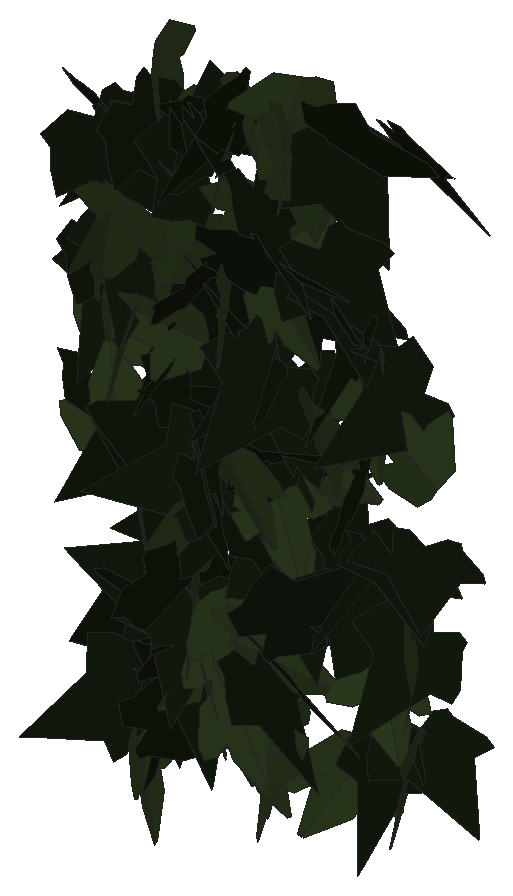
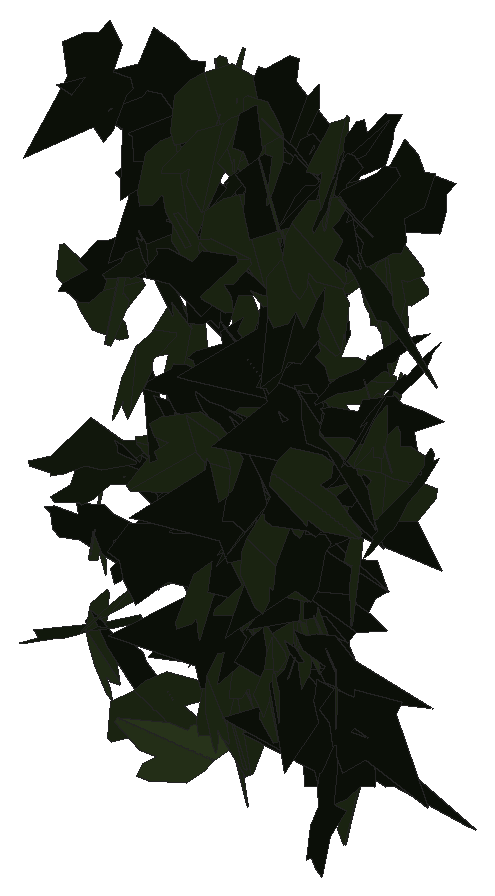
# SketchUp Ruby script. Lengths in inches.
U = 1.inch
M = Sketchup.active_model
def pt(a) = Geom::Point3d.new(a.map { |v| v * U })
def face(e, loops, mat)
  f = e.add_face(loops[0].map { |a| pt(a) })
  loops[1..].each { |l| e.add_face(l.map { |a| pt(a) }).erase! }
  f.material = f.back_material = mat if mat
  f
end
# faces: each face lists its corners as indices into pts; further lists are holes
def faces(e, pts, list, mat = nil) = list.each { |f| face(e, (f[0].is_a?(Array) ? f : [f]).map { |l| l.map { |i| pts[i] } }, mat) }
# xy, xz, yz: faces in a plane at the given z, y or x. An outline is a flat list of corners, or four numbers for a rectangle; further outlines are holes
def ring(l) = l.size == 4 ? [[l[0], l[1]], [l[2], l[1]], [l[2], l[3]], [l[0], l[3]]] : l.each_slice(2).to_a
def flat(e, list, mat, &to3) = list.each { |f| face(e, (f[0].is_a?(Array) ? f : [f]).map { |l| ring(l).map { |u, v| to3.(u, v) } }, mat) }
def xy(e, z, list, mat = nil) = flat(e, list, mat) { |x, y| [x, y, z] }
def xz(e, y, list, mat = nil) = flat(e, list, mat) { |x, z| [x, y, z] }
def yz(e, x, list, mat = nil) = flat(e, list, mat) { |y, z| [x, y, z] }
def lines(e, pts, list) = list.each { |a, b| e.add_line(pt(pts[a]), pt(pts[b])) }
# prism: a flat outline (further loops are holes) pulled along v
def prism(e, loops, v, mat = nil)
  f = face(e, loops, mat); d = Geom::Vector3d.new(v.map { |x| x * U })
  f.pushpull(f.normal.samedirection?(d) ? d.length : -d.length)
end
def box(e, o, s, mat = nil) = prism(e, [[o, [o[0] + s[0], o[1], o[2]], [o[0] + s[0], o[1] + s[1], o[2]], [o[0], o[1] + s[1], o[2]]]], [0, 0, s[2]], mat)
def at(x, y, z, deg = 0) = Geom::Transformation.translation(pt([x, y, z])) * Geom::Transformation.rotation(ORIGIN, Z_AXIS, deg.degrees)
def axes(o, x, y, z) = Geom::Transformation.new([*x, 0, *y, 0, *z, 0, *pt(o).to_a, 1])
def part(name) = M.definitions.add(name)
# library, detail: a bought-in or finely detailed component or shape, given as its bounding box
def library(name, o, s) = part(name).tap { |d| box(d.entities, o, s) }
def detail(e, o, s) = box(e.add_group.entities, o, s)
def put(e, d, t, mat = nil) = e.add_instance(d, t).tap { |i| i.material = mat if mat }
def group(e, t, mat = nil) = e.add_group.tap { |g| g.transformation = t; g.material = mat if mat }.entities
root = M.entities
M.materials.add("efeu1").color = [18, 25, 13]
M.materials.add("efeu2").color = [43, 57, 29]
c1 = part("ivyleaf_9")
p = [[1.54,2.16,1.25],[1.36,2.04,1.19],[-0.21,0.99,0.68],[-0.71,1.11,0.82],[-0.85,0.86,0.67],[-0.8,0.17,0.21],
  [-0.9,-0.01,0.1],[-0.67,-0.16,-0.02],[-0.08,-0.08,-0.05],[-0.03,-0.6,-0.4],[0.65,-0.88,-0.66],[0.83,-0.6,-0.49],
  [1.29,-0.42,-0.43],[1.8125,-0.07,-0.26],[1.21,0.44,0.15]]
faces(c1.entities,p,[[0,1,2,3,4,5,6,7,8,9,10,11,12,13,14]],"efeu1")
c2 = part("ivyleaf_10")
p = [[0,0.5,-0.03],[-0.0625,2.02,-0.43],[-0.19,2.01,-0.46],[-0.54,1.05,-0.29],[-0.52,0.625,-0.18],[-0.83,0.76,-0.28],
  [-1.16,0.64,-0.33],[-1.15,0.33,-0.24],[-0.77,-0.39,0.02],[-0.3,-0.51,0.16],[0.04,-0.48,0.23],[-0.02,2.01,-0.4375],
  [-0.06,2.01,-0.43],[0.04,-0.49,0.23],[0.67,-0.49,0.14],[1.38,0.36,-0.2],[1.375,0.51,-0.24],[0.81,0.65,-0.19],
  [0.62,0.59,-0.15],[0.6,1.09,-0.28],[0.5,1.23,-0.31]]
faces(c2.entities,p,[[0,1,2,3,4,5,6,7,8,9,10],[11,12,0,13,14,15,16,17,18,19,20]],"efeu2")
put(root,c1,axes([46.8,220.97,240.32],[0.3865,-0.05455,0.31248],[0.31369,-0.00741,-0.38929],[0.0471,0.49696,0.0285]))
put(root,c1,axes([46.45,221.32,237.34],[-0.37233,-0.02297,0.33293],[-0.32073,-0.11324,-0.36649],[0.09223,-0.48647,0.06959]))
put(root,c2,axes([45.4,221.08,240.3],[-0.46109,-0.04072,0.18904],[-0.18522,-0.04747,-0.462],[0.05558,-0.49607,0.02869]))
put(root,c1,axes([47.14,221.15,235.26],[0.24333,-0.42307,-0.10864],[-0.00438,0.12198,-0.48487],[0.43677,0.23692,0.05565]))
put(root,c1,axes([47.59,220.82,236.08],[0.04335,-0.00485,0.49809],[0.43952,0.23565,-0.03596],[-0.23441,0.44096,0.02469]))
put(root,c2,axes([46.95,221.07,237.77],[-0.45451,0.15093,-0.14368],[0.13832,-0.03931,-0.47887],[-0.15585,-0.47505,-0.00602]))
put(root,c1,axes([45.6,220.99,241.68],[0.15793,-0.2727,-0.38819],[-0.19318,0.33671,-0.31513],[0.43329,0.24952,0.001]))
put(root,c2,axes([46.45,221.12,235.07],[-0.28638,0.40461,-0.06538],[0.04195,-0.0504,-0.49568],[-0.40771,-0.28939,-0.00508]))
put(root,c2,axes([45.11,221.16,240.08],[0.05069,-0.48393,-0.11506],[-0.00378,0.11528,-0.48651],[0.49741,0.05019,0.00802]))
put(root,c2,axes([47.09,221.34,234.12],[0.22014,-0.15433,-0.42157],[0.35015,-0.23481,0.26881],[-0.28095,-0.41358,0.0047]))
put(root,c1,axes([46.64,221.52,241.95],[-0.16242,0.05528,-0.46964],[0.24306,-0.4162,-0.13305],[-0.40563,-0.27152,0.10833]))
put(root,c2,axes([46.91,221.08,234.8],[0.20428,0.43228,0.14629],[0.06712,0.13007,-0.4781],[-0.4514,0.21497,-0.00489]))
put(root,c1,axes([47.12,221.55,238.77],[-0.27886,-0.37937,0.16826],[-0.10219,-0.13371,-0.47083],[0.40224,-0.29698,-0.00296]))
put(root,c1,axes([46.08,221.39,235.74],[-0.32828,-0.32936,-0.18372],[0.13373,0.12609,-0.46499],[0.35263,-0.35444,0.00531]))
put(root,c2,axes([46.48,221.46,239.78],[0.21073,-0.29148,0.34732],[0.2627,-0.23369,-0.3555],[0.36957,0.33231,0.05465]))
put(root,c1,axes([48.99,221.6,239.09],[-0.26032,-0.30662,0.29702],[-0.19163,-0.22693,-0.40222],[0.38146,-0.32325,0.00064]))
put(root,c1,axes([46.98,221.33,240.98],[0.28987,-0.40717,-0.01377],[-0.00797,0.01123,-0.49981],[0.40732,0.28998,0.00001]))
put(root,c1,axes([45,221.09,241.28],[-0.0026,-0.26845,-0.42182],[0.01219,0.42166,-0.26842],[0.49984,-0.01168,0.00435]))
put(root,c2,axes([45.51,221.24,233.6875],[-0.13103,0.47752,-0.0693],[0.01853,-0.06678,-0.49517],[-0.48217,-0.13234,-0.0002]))
put(root,c2,axes([49.36,221.24,238.45],[0.27981,0.08174,0.40623],[-0.40276,-0.06157,0.28982],[0.0974,-0.48942,0.03139]))
put(root,c1,axes([45.51,221.43,237.51],[0.04991,0.09928,-0.48749],[-0.23004,-0.42982,-0.11109],[-0.44113,0.23537,0.00277]))
put(root,c2,axes([45.97,221.55,235.625],[0.18684,-0.17763,0.42842],[0.31477,-0.29063,-0.25778],[0.3406,0.36603,0.00322]))
put(root,c2,axes([46.27,221.24,236.95],[-0.11995,-0.47387,-0.10515],[0.02458,0.10224,-0.48882],[0.48478,-0.12244,-0.00123]))
put(root,c1,axes([45.9,220.89,236.13],[-0.01835,0.1511,-0.47627],[-0.10473,0.46484,0.15151],[0.48856,0.10532,0.01459]))
put(root,c2,axes([47.08,221.33,234.27],[-0.44844,0.04095,-0.21731],[-0.21722,0.01045,0.45023],[0.04141,0.49821,0.00842]))
put(root,c2,axes([45.18,221.39,238.78],[0.28611,-0.40895,0.03005],[0.01789,-0.02416,-0.4991],[0.40966,0.28667,0.0008]))
put(root,c1,axes([46,221.41,237.5625],[-0.13717,-0.06246,-0.47674],[0.46737,0.09909,-0.14746],[0.1129,-0.48609,0.0312]))
put(root,c1,axes([46.26,221.26,241.59],[0.42677,-0.24662,-0.08393],[-0.06824,0.04963,-0.49283],[0.25142,0.4321,0.0087]))
put(root,c1,axes([44.72,221.45,241.19],[0.27844,-0.27235,0.31351],[0.2605,-0.17942,-0.38723],[0.32343,0.37899,0.04198]))
put(root,c2,axes([47.47,221.17,241.82],[0.25936,-0.28035,-0.32271],[-0.15566,0.2896,-0.37669],[0.39812,0.29586,0.06294]))
put(root,c1,axes([46.25,221.24,237.4375],[0.31981,-0.27864,-0.26473],[-0.1758,0.2002,-0.4231],[0.34178,0.3637,0.03009]))
put(root,c2,axes([46.64,221.31,235.36],[0.32468,0.37426,0.06716],[0.04255,0.05199,-0.49547],[-0.37785,0.32745,0.00191]))
put(root,c1,axes([46.01,221.61,240.8],[-0.04527,-0.4943,-0.06015],[0.05638,-0.0651,0.49253],[-0.49474,0.03781,0.06163]))
put(root,c2,axes([46.62,221.31,235.74],[0.20407,0.45593,0.02201],[0.01219,0.01865,-0.4995],[-0.4563,0.2044,-0.0035]))
put(root,c1,axes([45.18,221.47,234.19],[-0.46648,0.07003,0.16582],[-0.16471,0.01968,-0.47168],[-0.07259,-0.49468,0.00471]))
put(root,c2,axes([46.28,221.6875,235.01],[0.01666,0.21113,-0.45293],[-0.1853,-0.41826,-0.20179],[-0.4641,0.17458,0.06431]))
put(root,c1,axes([46.01,221.47,234.94],[-0.28027,-0.15592,-0.38358],[0.34576,0.16671,-0.3204],[0.22781,-0.44486,0.01437]))
put(root,c1,axes([46.38,221.38,236.81],[-0.40019,0.19108,0.23094],[-0.21769,0.07954,-0.44304],[-0.20605,-0.45515,0.01953]))
put(root,c1,axes([45.76,221.09,234.12],[0.15187,0.07913,0.46976],[0.4243,0.2017,-0.17115],[-0.21658,0.45062,-0.00588]))
put(root,c2,axes([47.89,221.31,238.53],[-0.46044,0.18598,0.05835],[-0.05402,0.02207,-0.49658],[-0.18729,-0.4636,-0.00023]))
put(root,c2,axes([47.25,221.58,241.38],[-0.2165,0.36448,0.26511],[0.12921,-0.23157,0.42389],[0.43178,0.25205,0.00608]))
put(root,c2,axes([47.05,221.61,235.58],[-0.23287,-0.32846,0.29645],[-0.16387,-0.24715,-0.40257],[0.41099,-0.28465,0.00746]))
put(root,c2,axes([45.04,221.35,237.36],[0.38861,0.31443,0.01081],[-0.01058,-0.0041,0.49987],[0.31443,-0.38874,0.00347]))
put(root,c2,axes([45.47,221.26,236.81],[-0.23988,0.38309,0.21378],[-0.18833,0.13013,-0.44452],[-0.39622,-0.29378,0.08186]))
put(root,c2,axes([46.98,221.4,235.37],[-0.16905,0.01972,-0.47014],[0.47032,-0.00867,-0.16948],[-0.01484,-0.49954,-0.01562]))
put(root,c1,axes([47.02,221.46,235.25],[0.4307,-0.21881,0.12891],[0.11656,-0.05517,-0.48308],[0.22563,0.44618,0.00348]))
put(root,c1,axes([44.51,221.64,237.69],[0.22848,-0.43045,0.11183],[0.06616,-0.09143,-0.4871],[0.43979,0.23738,0.01518]))
put(root,c2,axes([47.12,221.45,237.28],[0.43584,0.12416,0.21125],[0.20167,0.06311,-0.45315],[-0.13919,0.48021,0.00494]))
put(root,c2,axes([46.28,221.4,235.5],[-0.48934,0.05727,0.08524],[-0.08591,-0.00088,-0.49256],[-0.05627,-0.49671,0.0107]))
put(root,c2,axes([45.98,221.6,240.08],[-0.24076,-0.39503,0.18971],[-0.10624,-0.15739,-0.46254],[0.42515,-0.26303,-0.00815]))
put(root,c2,axes([47.09,221.52,233.97],[0.33007,-0.37391,-0.03533],[-0.00901,0.03914,-0.49838],[0.37546,0.32964,0.0191]))
put(root,c1,axes([47.02,221.53,238.86],[-0.45965,0.19027,-0.05021],[0.04713,-0.01742,-0.49747],[-0.19105,-0.46206,-0.00192]))
put(root,c2,axes([45.86,221.5,238.78],[-0.08838,0.00362,-0.49211],[-0.49051,0.03991,0.08838],[0.03992,0.49839,-0.0035]))
put(root,c1,axes([46.21,221.11,239.66],[0.15741,0.43259,0.19515],[0.0444,0.19128,-0.45983],[-0.47249,0.1621,0.02181]))
put(root,c1,axes([48.2,221.62,239.65],[-0.39666,0.1439,-0.26824],[0.24774,-0.10338,-0.42182],[-0.17686,-0.46755,0.01072]))
put(root,c1,axes([46.3,221.4,241.39],[-0.31342,0.2725,0.27841],[-0.22956,0.15952,-0.41456],[-0.31476,-0.38768,0.02512]))
put(root,c1,axes([46.12,221.27,235.16],[0.19447,0.45928,-0.03522],[-0.01608,-0.03144,-0.49875],[-0.46035,0.19511,0.00254]))
put(root,c1,axes([45.9,221.51,237.98],[0.07285,0.04347,-0.49275],[-0.44488,-0.21199,-0.08448],[-0.21627,0.45074,0.00779]))
put(root,c1,axes([47.82,221.42,240.49],[-0.10976,-0.17576,-0.45504],[0.21861,0.39924,-0.20693],[0.43608,-0.24438,-0.0108]))
put(root,c1,axes([46.64,221.6,236.85],[0.29263,-0.40409,-0.03291],[-0.00048,0.04024,-0.49838],[0.40542,0.29171,0.02316]))
put(root,c2,axes([48.76,221.8,234.53],[0.24445,-0.31746,0.2991],[0.1763,-0.24171,-0.40062],[0.39895,0.30132,-0.00623]))
put(root,c2,axes([49.16,221.22,235.8],[0.01221,-0.03848,-0.49837],[-0.16311,0.47092,-0.04035],[0.47249,0.16356,-0.00105]))
put(root,c1,axes([47.83,221.86,239.79],[-0.01841,-0.46428,0.18468],[0.23969,-0.17036,-0.40438],[0.43842,0.07364,0.22884]))
put(root,c2,axes([46.91,221.63,234.49],[-0.20998,-0.45109,0.04926],[-0.01962,-0.0452,-0.49757],[0.45335,-0.21089,0.00128]))
put(root,c1,axes([48.51,221.75,234.6],[-0.40094,-0.08354,-0.28682],[0.28881,0.01435,-0.4079],[0.07638,-0.49276,0.03675]))
put(root,c1,axes([48.95,221.82,236.03],[-0.46699,-0.17498,-0.036],[0.03535,0.00825,-0.49868],[0.17512,-0.46831,0.00466]))
put(root,c2,axes([45.36,221.9,235.4],[-0.18244,0.09592,-0.45554],[0.19412,-0.42903,-0.16809],[-0.42312,-0.23819,0.1193]))
put(root,c2,axes([46.88,221.66,239.62],[0.25686,-0.05482,0.42546],[0.42879,0.01809,-0.25654],[0.01274,0.49666,0.05631]))
put(root,c1,axes([47.2,221.75,239.76],[0.22886,-0.11332,-0.42986],[0.44358,0.09008,0.21242],[0.0293,-0.47859,0.14177]))
put(root,c2,axes([48.27,221.86,235.27],[-0.21667,-0.43016,0.13422],[0.36917,-0.25485,-0.22083],[0.25839,0.0034,0.42804]))
put(root,c1,axes([45.55,221.99,241.07],[-0.04965,-0.16868,0.46806],[0.07101,-0.46797,-0.16112],[0.49244,0.05047,0.07043]))
put(root,c1,axes([48.08,221.99,236.02],[-0.0507,-0.40479,-0.28909],[0.0046,-0.29096,0.4066],[-0.4974,0.03856,0.03323]))
put(root,c1,axes([45.9375,221.95,239.1875],[0.01465,-0.28899,0.40776],[0.21881,-0.36306,-0.26517],[0.44934,0.18621,0.11583]))
put(root,c1,axes([48.45,221.95,236.73],[-0.01828,-0.46971,0.1704],[0.27755,-0.15133,-0.38738],[0.41549,0.08043,0.26627]))
put(root,c2,axes([46.35,221.76,241.73],[-0.27755,0.21723,-0.35465],[0.27793,-0.2203,-0.35245],[-0.30939,-0.39278,0.00154]))
put(root,c1,axes([45.69,221.54,238.4375],[-0.26839,0.42151,0.01729],[-0.00996,0.01416,-0.4997],[-0.42174,-0.26858,0.00079]))
put(root,c2,axes([47.2,221.59,236],[0.49499,0.0437,0.05548],[-0.05716,0.01728,0.49642],[0.04147,-0.49779,0.02211]))
put(root,c2,axes([47.14,221.8,242.04],[-0.26381,-0.40149,0.1386],[-0.01366,-0.15505,-0.47516],[0.42452,-0.25449,0.07084]))
put(root,c1,axes([45.33,221.59,234.43],[0.1307,0.09798,-0.47256],[0.40254,0.24794,0.16274],[0.26623,-0.42299,-0.01407]))
put(root,c1,axes([47.15,221.79,236.49],[-0.12447,-0.42735,-0.22776],[0.10507,0.20573,-0.44344],[0.47272,-0.15826,0.03859]))
put(root,c1,axes([47.11,221.66,237.76],[-0.37997,0.17262,0.27536],[-0.24693,0.12209,-0.41728],[-0.2113,-0.4531,-0.00753]))
put(root,c1,axes([46.04,221.71,241.44],[0.01586,0.32813,-0.37694],[-0.20208,-0.34071,-0.30509],[-0.45707,0.16202,0.12181]))
put(root,c1,axes([48.05,221.86,237.01],[-0.45307,-0.05181,-0.20504],[0.20502,0.01128,-0.45589],[0.05187,-0.49718,0.01102]))
put(root,c1,axes([46.65,221.63,237.3],[0.36775,0.24688,-0.23197],[0.19482,0.12596,0.44292],[0.27713,-0.41616,-0.00355]))
put(root,c2,axes([46.72,221.75,240.59],[-0.40889,-0.2276,0.17607],[-0.14939,-0.09359,-0.46789],[0.24594,-0.43525,0.00853]))
put(root,c1,axes([48.71,222.04,236.91],[-0.15357,-0.46768,0.08769],[0.29983,-0.16665,-0.36377],[0.36948,-0.05914,0.33164]))
put(root,c1,axes([48.23,221.34,237.47],[-0.04458,0.24016,0.43627],[-0.06106,0.43208,-0.24409],[-0.49425,-0.07504,-0.0092]))
put(root,c2,axes([46.28,221.83,241.3],[0.26633,-0.42131,0.03957],[0.01733,-0.03586,-0.49841],[0.42281,0.26685,-0.0045]))
put(root,c1,axes([44.8125,222.03,239.48],[-0.08445,-0.48592,0.08216],[0.03471,-0.08902,-0.49079],[0.49159,-0.07719,0.04877]))
put(root,c1,axes([45.13,221.71,234.97],[0.02927,0.09947,-0.48913],[-0.44745,-0.21191,-0.06987],[-0.22121,0.44181,0.07661]))
put(root,c2,axes([48.46,221.875,238.73],[-0.31226,0.32214,0.22073],[0.15627,-0.15593,0.44863],[0.35787,0.34916,-0.0033]))
put(root,c2,axes([47.94,221.91,234.1],[0.33088,0.23904,-0.28876],[-0.23553,-0.16706,-0.40819],[-0.29163,0.40614,0.00205]))
put(root,c2,axes([46.62,221.68,235.08],[-0.37315,0.08014,0.32301],[-0.31959,0.04913,-0.38138],[-0.09286,-0.49109,0.01456]))
put(root,c1,axes([48.76,221.95,234.72],[0.05901,-0.49003,-0.07991],[0.27559,0.09926,-0.40521],[0.413,0.00378,0.28181]))
put(root,c2,axes([45.48,221.63,241.97],[-0.14217,0.44948,0.16661],[-0.13757,0.12822,-0.46329],[-0.4592,-0.17757,0.08721]))
put(root,c1,axes([44.41,221.77,239.36],[0.25601,-0.36645,-0.224],[-0.09215,0.20784,-0.44532],[0.41948,0.2693,0.03888]))
put(root,c1,axes([45.56,221.8,237.46],[0.01262,-0.07899,0.49356],[0.47745,-0.14422,-0.03529],[0.14794,0.47219,0.07179]))
put(root,c1,axes([47.68,221.77,241.68],[0.30436,-0.06779,0.39086],[0.37848,-0.09795,-0.31171],[0.11883,0.4856,-0.00831]))
put(root,c1,axes([47.07,221.95,238.52],[-0.21686,-0.36842,-0.2593],[0.17041,0.19932,-0.42572],[0.41706,-0.27301,0.03911]))
put(root,c1,axes([45.93,221.57,239.03],[0.32808,0.10707,0.3618],[0.34555,0.1073,-0.34509],[-0.15154,0.47647,-0.00359]))
put(root,c2,axes([47.17,221.79,235.83],[-0.08559,0.4926,0.00433],[-0.14891,-0.02168,-0.47682],[-0.46957,-0.08292,0.15042]))
put(root,c1,axes([47.68,221.8,241.59],[-0.14613,-0.27578,-0.39063],[0.16572,0.35393,-0.31188],[0.44853,-0.22062,-0.01203]))
put(root,c2,axes([44.52,221.9375,239.02],[-0.07175,0.45038,-0.20496],[0.0406,-0.20104,-0.456],[-0.49316,-0.08208,-0.00772]))
put(root,c2,axes([44.75,221.78,238.23],[0.48013,0.13524,0.03445],[-0.03803,0.00804,0.49849],[0.13428,-0.48129,0.01801]))
put(root,c1,axes([45.43,221.82,235.36],[-0.26083,0.16431,0.39366],[-0.3673,0.14815,-0.3052],[-0.21694,-0.44839,0.04341]))
put(root,c2,axes([46.1,222.19,236.76],[0.03399,-0.38036,0.32275],[0.0316,-0.32121,-0.38187],[0.49784,0.04636,0.0022]))
put(root,c1,axes([45.21,222.26,233.86],[-0.01378,-0.0969,-0.49033],[0.40421,-0.29067,0.04608],[-0.29398,-0.39512,0.08634]))
put(root,c2,axes([47.0625,221.95,237.4375],[-0.05719,0.02067,-0.49629],[0.48319,-0.11349,-0.06041],[-0.11514,-0.48651,-0.007]))
put(root,c2,axes([47.01,221.86,241.55],[0.09011,0.49134,0.02157],[0.00319,0.02134,-0.49953],[-0.4918,0.09016,0.00071]))
put(root,c2,axes([47.46,221.98,241.19],[-0.21573,-0.44881,0.04504],[-0.01036,-0.04499,-0.49786],[0.45095,-0.21574,0.01011]))
put(root,c1,axes([44.7,222.17,239],[-0.38007,-0.32189,-0.0439],[0.0343,0.02743,-0.49807],[0.32306,-0.38162,0.00123]))
put(root,c2,axes([46.79,222.15,234.73],[0.15416,-0.40223,0.25387],[0.16816,-0.20354,-0.42461],[0.44492,0.2163,0.07252]))
put(root,c1,axes([45.86,221.79,236.86],[0.49223,0.01048,-0.08716],[-0.08727,0.00445,-0.49231],[-0.00954,0.49987,0.00621]))
put(root,c1,axes([46.67,221.62,236.99],[0.25031,0.14145,0.40907],[0.33194,0.24054,-0.28629],[-0.27778,0.41489,0.02651]))
put(root,c2,axes([45.44,222.25,241.02],[-0.00008,-0.3933,0.30874],[0.06975,-0.30573,-0.38944],[0.49511,0.04301,0.05491]))
put(root,c1,axes([45.58,221.89,238.41],[0.07192,-0.08558,-0.48734],[0.35474,0.35223,-0.0095],[0.34494,-0.3444,0.11139]))
put(root,c1,axes([44.78,221.99,240.64],[-0.40523,0.2901,-0.04043],[0.03306,-0.02328,-0.49836],[-0.29103,-0.40657,-0.00031]))
put(root,c2,axes([45.84,221.97,237.63],[0.17526,-0.03335,-0.46709],[-0.45119,0.12146,-0.17797],[0.12534,0.48387,0.01248]))
put(root,c2,axes([47.87,222.18,238.54],[0.01223,-0.46696,0.17831],[0.2713,-0.14361,-0.39468],[0.41982,0.1064,0.24986]))
put(root,c2,axes([47.18,222.05,233.73],[0.01336,-0.49522,0.06766],[0.46662,0.03662,0.17585],[-0.17912,0.05844,0.46314]))
put(root,c1,axes([47.0625,222.1875,240.08],[-0.36873,-0.28367,-0.18322],[0.13988,0.11861,-0.46515],[0.30736,-0.39429,-0.00811]))
put(root,c1,axes([47.52,222.25,236.6],[-0.052,0.17847,-0.46416],[-0.0019,-0.46676,-0.17926],[-0.49728,-0.01688,0.04922]))
put(root,c2,axes([47.13,221.89,237.61],[-0.28168,-0.10569,-0.39936],[0.37631,0.13376,-0.30083],[0.17042,-0.47004,0.00419]))
put(root,c1,axes([46.9,221.7,235.31],[0.20156,0.12891,0.43904],[0.37241,0.23253,-0.23924],[-0.26586,0.42345,-0.00228]))
put(root,c2,axes([47.19,221.98,239.93],[0.2575,0.05254,0.42537],[-0.427,-0.01133,0.25989],[0.03695,-0.4971,0.03903]))
put(root,c1,axes([48.47,221.95,241.9],[0.4926,-0.08171,-0.02587],[-0.02525,0.00588,-0.49933],[0.0819,0.49324,0.00167]))
